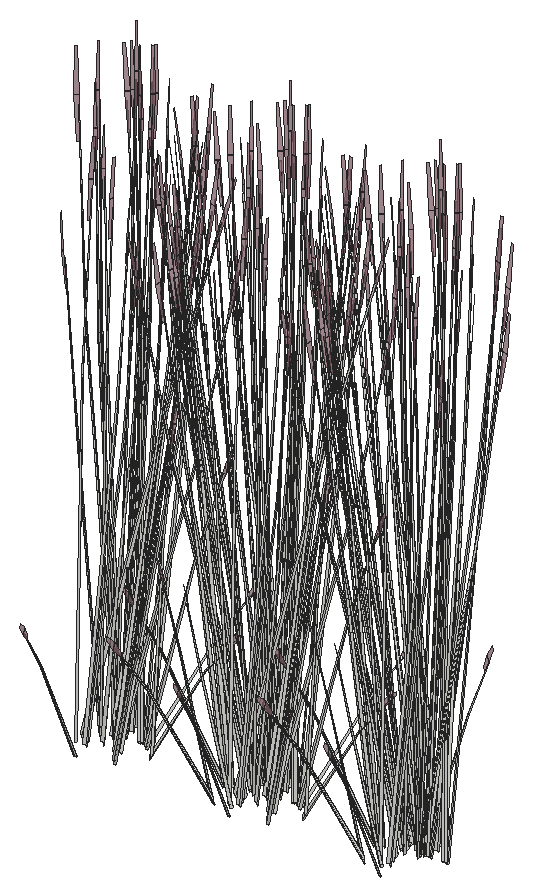
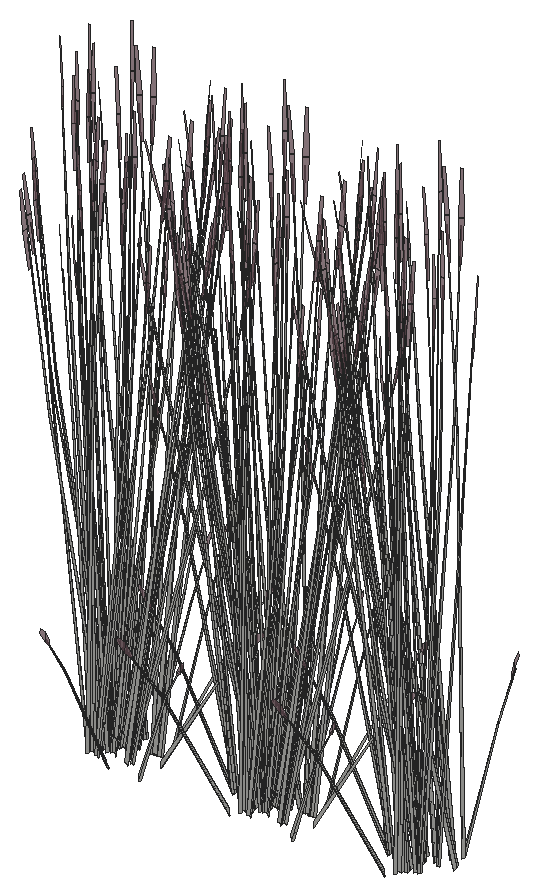
# SketchUp Ruby script. Lengths in inches.
U = 1.inch
M = Sketchup.active_model
def pt(a) = Geom::Point3d.new(a.map { |v| v * U })
def face(e, loops, mat)
  f = e.add_face(loops[0].map { |a| pt(a) })
  loops[1..].each { |l| e.add_face(l.map { |a| pt(a) }).erase! }
  f.material = f.back_material = mat if mat
  f
end
# faces: each face lists its corners as indices into pts; further lists are holes
def faces(e, pts, list, mat = nil) = list.each { |f| face(e, (f[0].is_a?(Array) ? f : [f]).map { |l| l.map { |i| pts[i] } }, mat) }
# xy, xz, yz: faces in a plane at the given z, y or x. An outline is a flat list of corners, or four numbers for a rectangle; further outlines are holes
def ring(l) = l.size == 4 ? [[l[0], l[1]], [l[2], l[1]], [l[2], l[3]], [l[0], l[3]]] : l.each_slice(2).to_a
def flat(e, list, mat, &to3) = list.each { |f| face(e, (f[0].is_a?(Array) ? f : [f]).map { |l| ring(l).map { |u, v| to3.(u, v) } }, mat) }
def xy(e, z, list, mat = nil) = flat(e, list, mat) { |x, y| [x, y, z] }
def xz(e, y, list, mat = nil) = flat(e, list, mat) { |x, z| [x, y, z] }
def yz(e, x, list, mat = nil) = flat(e, list, mat) { |y, z| [x, y, z] }
def lines(e, pts, list) = list.each { |a, b| e.add_line(pt(pts[a]), pt(pts[b])) }
# prism: a flat outline (further loops are holes) pulled along v
def prism(e, loops, v, mat = nil)
  f = face(e, loops, mat); d = Geom::Vector3d.new(v.map { |x| x * U })
  f.pushpull(f.normal.samedirection?(d) ? d.length : -d.length)
end
def box(e, o, s, mat = nil) = prism(e, [[o, [o[0] + s[0], o[1], o[2]], [o[0] + s[0], o[1] + s[1], o[2]], [o[0], o[1] + s[1], o[2]]]], [0, 0, s[2]], mat)
def at(x, y, z, deg = 0) = Geom::Transformation.translation(pt([x, y, z])) * Geom::Transformation.rotation(ORIGIN, Z_AXIS, deg.degrees)
def axes(o, x, y, z) = Geom::Transformation.new([*x, 0, *y, 0, *z, 0, *pt(o).to_a, 1])
def part(name) = M.definitions.add(name)
# library, detail: a bought-in or finely detailed component or shape, given as its bounding box
def library(name, o, s) = part(name).tap { |d| box(d.entities, o, s) }
def detail(e, o, s) = box(e.add_group.entities, o, s)
def put(e, d, t, mat = nil) = e.add_instance(d, t).tap { |i| i.material = mat if mat }
def group(e, t, mat = nil) = e.add_group.tap { |g| g.transformation = t; g.material = mat if mat }.entities
root = M.entities
M.materials.add("LightPink_Translucent").color = [144, 107, 117]
M.materials["LightPink_Translucent"].alpha = 0.75
c1 = part("blade")
p = [[2.15,0.21,22],[0,0.17,0],[0.09,0.45,0],[2.18,0.31,22],[2.29,0.31,22],[0.38,0.45,0],
  [2.48,0.24,33],[2.49,0.24,33],[2.48,0.22,33]]
faces(c1.entities,p,[[0,1,2,3],[4,5,2,3],[6,3,4,7],[8,0,3,6]])
c2 = part("seeds")
p = [[0.3,-0.1,1.38],[-0.01,-0.03,1.59],[-0.01,-0.03,0.03],[0.14,-0.07,-0.07],[0.29,-0.03,3],[0.15,0.01,3.11]]
faces(c2.entities,p,[[0,1,2,3],[1,0,4,5]],"LightPink_Translucent")
c3 = part("blade with seeds")
put(c3.entities,c1,at(0,0,0))
put(c3.entities,c2,axes([2.4,0.25,30.99],[1.5799,-0.05474,1.17369],[-0.12525,1.92788,0.29478],[-0.07173,-0.02425,1.56792]))
put(root,c3,axes([278.62,55.33,257.2],[-0.76598,-0.27433,0],[0.36864,-0.57001,0],[0,0,1.62707]))
put(root,c3,axes([280.39,56.02,257.375],[0.47504,0.61229,0],[-0.79476,0.34146,-0.51607],[-0.18101,0.07777,1.63711]))
put(root,c3,axes([279.42,54.01,257.3],[-0.70674,-0.52593,-0.06131],[0.70717,-0.52625,0],[-0.02468,-0.01837,1.75571]))
put(root,c3,axes([279.8125,55.63,257.33],[0.95122,0.19861,0.30756],[-0.23797,0.7099,-0.36492],[-0.15744,0.08885,1.64885]))
put(root,c3,axes([278.42,50.1875,256.49],[-0.12744,0.02202,1.76342],[-0.70477,-0.24781,-0.26939],[0.01183,-0.2067,0.30037]))
put(root,c3,axes([277.85,53.32,257.21],[0.36864,-0.55059,-0.44739],[0.76598,0.26498,0.21531],[0,-0.12692,1.43643]))
put(root,c3,axes([278.79,55.09,257.2],[-0.24791,-0.5268,0],[0.70791,-0.18448,0],[0,0,1.54371]))
put(root,c3,axes([279.79,54.05,257.21],[-0.36864,0.55059,-0.44739],[-0.76598,-0.26498,0.21531],[0,0.12692,1.43643]))
put(root,c3,axes([279.1875,53.46,257.21],[0,-0.70701,0],[0.95008,0,0],[0,0,1.79456]))
put(root,c3,axes([279.66,53.74,257.29],[0,0.70667,-0.05637],[-0.95008,0,0],[0,0.02221,1.79368]))
put(root,c3,axes([279.21,55.11,257.29],[0.33034,0.70197,-0.06012],[-0.94388,0.24598,0],[0.01154,0.02451,1.72173]))
put(root,c3,axes([277.25,51.35,257.375],[-0.47504,-0.61229,0],[0.79476,-0.34146,-0.51607],[0.18101,-0.07777,1.63711]))
put(root,c3,axes([281.9375,54.19,257.2],[-0.94962,-0.00489,-0.04976],[0,-0.68292,0.49943],[-0.02984,0.15546,1.58352]))
put(root,c3,axes([279.8125,53.89,257.21],[0.53038,0.39469,0],[-0.53038,0.39469,0],[0,0,1.69266]))
put(root,c3,axes([279.49,55.34,257.2],[0.76598,0.27433,0],[-0.36864,0.57001,0],[0,0,1.74954]))
put(root,c3,axes([281.74,54.29,257.03],[-0.53038,0.38124,-0.30978],[-0.53038,-0.38124,0.30978],[0,0.1228,1.38974]))
put(root,c3,axes([280.23,54.22,257.09],[0.2786,0.55945,-0.69212],[-0.80253,0.20149,-0.18165],[0.03079,0.18945,1.52773]))
put(root,c3,axes([279.83,53.62,257.21],[0.85008,0,0],[0,0.63259,0],[0,0,1.78407]))
put(root,c3,axes([278.18,53.04,257.67],[-0.08854,-0.69723,-0.29095],[0.92215,-0.04216,-0.50002],[0.16238,-0.09287,1.59708]))
put(root,c3,axes([279.88,53.6,257.67],[0.85568,0.29155,-0.29095],[-0.41201,0.61537,-0.50002],[0.02689,0.15109,1.59708]))
put(root,c3,axes([278.0625,51.5,257.03],[0.70886,0.15119,-0.30978],[-0.17848,0.53243,0.30978],[0.1429,-0.0614,1.38974]))
put(root,c3,axes([282.11,54.3,257.02],[0,0.61104,-0.49651],[-0.85008,0,0],[0,0.13917,1.57504]))
put(root,c3,axes([277.9,51.26,257.02],[0.7111,-0.30552,-0.49651],[0.42504,0.54784,0],[0.16196,-0.06958,1.57504]))
put(root,c3,axes([279.72,55.02,257.18],[0.79769,-0.20732,-0.19198],[0.2803,0.59721,0.00008],[0.08805,-0.02292,1.73897]))
put(root,c3,axes([279.73,53.24,257.21],[0.45644,0.51287,-0.44739],[-0.69137,0.36116,0.21531],[0.14771,0.06346,1.43643]))
put(root,c3,axes([278.74,52.51,257.06],[0.51177,-0.45928,-0.62353],[0.63575,0.41646,-0.16365],[0.20507,-0.11457,1.37633]))
put(root,c3,axes([280.98,52.1,257.03],[0.17848,0.53243,-0.30978],[-0.70886,0.15119,0.30978],[0.1429,0.0614,1.38974]))
put(root,c3,axes([282.32,53.84,257.375],[0.95008,0,0],[0,0.68292,-0.51607],[0,0.15554,1.63711]))
put(root,c3,axes([279.25,52.95,257.67],[0.76714,-0.40567,-0.29095],[0.51013,0.57321,-0.50002],[0.18927,0.05821,1.59708]))
put(root,c3,axes([277.3125,52.59,256.59],[-0.74787,0.24464,1.28929],[-0.23804,-0.70192,0.50096],[0.45924,0.01168,1.46642]))
put(root,c3,axes([280.75,51.51,257.375],[0.47504,-0.61229,0],[0.79476,0.34146,-0.51607],[0.18101,0.07777,1.63711]))
put(root,c3,axes([281.54,51.24,256.49],[-0.11372,-0.04814,1.76342],[-0.29211,-0.53779,-0.26939],[0.19706,-0.14594,0.30037]))
put(root,c3,axes([281.18,51.875,257.02],[0.7111,0.30552,-0.49651],[-0.42504,0.54784,0],[0.16196,0.06958,1.57504]))
put(root,c3,axes([281.15,56.22,256.49],[0.05536,-0.08822,1.76342],[0.69692,-0.25981,-0.26939],[0.21129,0.13447,0.30037]))
put(root,c3,axes([280.14,53.05,257.06],[0.79037,0.10018,-0.62353],[-0.16679,0.61794,-0.16365],[0.23587,0.07488,1.37633]))
put(root,c3,axes([283.51,53.41,257.26],[-0.47106,-0.39072,-0.06488],[0.51591,-0.35801,-0.29416],[0.14618,-0.02521,0.97024]))
put(root,c3,axes([290.68,53.45,256.49],[0.01927,0.0963,1.76342],[-0.38846,0.5029,-0.26939],[-0.27592,-0.02535,0.30037]))
put(root,c3,axes([290.47,56.15,256.49],[0.10192,0.06105,1.76342],[0.17281,0.56562,-0.26939],[-0.22588,0.12062,0.30037]))
put(root,c3,axes([293.22,54.32,257.06],[-0.79037,-0.10018,-0.62353],[0.16679,-0.61794,-0.16365],[-0.23587,-0.07488,1.37633]))
put(root,c3,axes([282.62,53.93,256.98],[-0.48937,0.07333,1.41583],[-0.07789,-0.58369,0.08104],[0.34275,-0.08835,0.80566]))
put(root,c3,axes([283.15,53.55,256.49],[-0.03971,-0.09277,1.76342],[0.27541,-0.54264,-0.26939],[0.27782,-0.00781,0.30037]))
put(root,c3,axes([292.1875,55.49,257.02],[-0.7111,-0.30552,-0.49651],[0.42504,-0.54784,0],[-0.16196,-0.06958,1.57504]))
put(root,c3,axes([291.875,50.94,256.49],[-0.0736,0.08049,1.76342],[-0.74378,0.17355,-0.26939],[-0.17968,-0.15788,0.30037]))
put(root,c3,axes([292.62,55.86,257.375],[-0.47504,0.61229,0],[-0.79476,-0.34146,-0.51607],[-0.18101,-0.07777,1.63711]))
put(root,c3,axes([291.41,51.25,257.13],[-0.21918,0.49894,-0.03893],[-0.6746,-0.15348,-0.17649],[-0.10242,-0.08161,0.58215]))
put(root,c3,axes([294.12,54.42,257.67],[-0.76714,0.40567,-0.29095],[-0.51013,-0.57321,-0.50002],[-0.18927,-0.05821,1.59708]))
put(root,c3,axes([291.05,53.53,257.375],[-0.95008,0,0],[0,-0.68292,-0.51607],[0,-0.15554,1.63711]))
put(root,c3,axes([292.38,55.27,257.03],[-0.17848,-0.53243,-0.30978],[0.70886,-0.15119,0.30978],[-0.1429,-0.0614,1.38974]))
put(root,c3,axes([294.63,54.86,257.06],[-0.51177,0.45928,-0.62353],[-0.63575,-0.41646,-0.16365],[-0.20507,0.11457,1.37633]))
put(root,c3,axes([291.79,53.35,257.33],[-0.70674,0.51372,0.30756],[-0.70717,-0.50832,-0.36492],[-0.02468,-0.14589,1.64885]))
put(root,c3,axes([294.98,54.6,257.46],[-0.74193,-0.49181,-0.25192],[0.6243,-0.55226,0.5513],[-0.19979,0.05753,1.68216]))
put(root,c3,axes([293.63,54.13,257.21],[-0.45644,-0.51287,-0.44739],[0.69137,-0.36116,0.21531],[-0.14771,-0.06346,1.43643]))
put(root,c3,axes([294.61,54.5,257.21],[-0.82508,0.03772,-0.44739],[-0.07462,-0.62614,0.21531],[-0.14771,0.06346,1.43643]))
put(root,c3,axes([293.7,54.42,257.4375],[0.20138,-0.72405,-0.23429],[0.95485,0.12621,0.51271],[-0.16685,-0.09999,1.5644]))
put(root,c3,axes([295.47,56.11,257.02],[-0.7111,0.30552,-0.49651],[-0.42504,-0.54784,0],[-0.16196,0.06958,1.57504]))
put(root,c3,axes([291.26,53.07,257.02],[0,-0.61104,-0.49651],[0.85008,0,0],[0,-0.13917,1.57504]))
put(root,c3,axes([295.52,55.95,257.19],[-0.46912,-0.61443,-0.05142],[0.79476,-0.34146,0.51607],[-0.19584,0.0585,1.6363]))
put(root,c3,axes([295.31,55.87,257.03],[-0.70886,-0.15119,-0.30978],[0.17848,-0.53243,0.30978],[-0.1429,0.0614,1.38974]))
put(root,c3,axes([293.48,53.77,257.67],[-0.85568,-0.29155,-0.29095],[0.41201,-0.61537,-0.50002],[-0.02689,-0.15109,1.59708]))
put(root,c3,axes([295.18,54.33,257.67],[0.08854,0.69723,-0.29095],[-0.92215,0.04216,-0.50002],[-0.16238,0.09287,1.59708]))
put(root,c3,axes([293.1,53.15,257.1],[-0.31203,-0.62659,-0.69835],[0.89884,-0.22566,-0.18329],[-0.03449,-0.21218,1.54149]))
put(root,c3,axes([291.625,53.08,257.03],[0.53038,-0.38124,-0.30978],[0.53038,0.38124,0.30978],[0,-0.1228,1.38974]))
put(root,c3,axes([294.02,50.62,257.13],[-0.52505,0.35054,-0.03893],[-0.48109,-0.38392,-0.17649],[-0.03387,-0.10878,0.58215]))
put(root,c3,axes([294.34,55.33,257.2],[-0.76598,-0.27433,0],[0.36864,-0.57001,0],[0,0,1.62707]))
put(root,c3,axes([296.12,56.02,257.375],[0.47504,0.61229,0],[-0.79476,0.34146,-0.51607],[-0.18101,0.07777,1.63711]))
put(root,c3,axes([295.15,54.01,257.3],[-0.70674,-0.52593,-0.06131],[0.70717,-0.52625,0],[-0.02468,-0.01837,1.75571]))
put(root,c3,axes([295.54,55.63,257.33],[0.95122,0.19861,0.30756],[-0.23797,0.7099,-0.36492],[-0.15744,0.08885,1.64885]))
put(root,c3,axes([294.15,50.1875,256.49],[-0.12744,0.02202,1.76342],[-0.70477,-0.24781,-0.26939],[0.01183,-0.2067,0.30037]))
put(root,c3,axes([293.58,53.32,257.21],[0.36864,-0.55059,-0.44739],[0.76598,0.26498,0.21531],[0,-0.12692,1.43643]))
put(root,c3,axes([294.52,55.09,257.2],[-0.24791,-0.5268,0],[0.70791,-0.18448,0],[0,0,1.54371]))
put(root,c3,axes([295.52,54.05,257.21],[-0.36864,0.55059,-0.44739],[-0.76598,-0.26498,0.21531],[0,0.12692,1.43643]))
put(root,c3,axes([294.92,53.46,257.21],[0,-0.70701,0],[0.95008,0,0],[0,0,1.79456]))
put(root,c3,axes([295.39,53.74,257.29],[0,0.70667,-0.05637],[-0.95008,0,0],[0,0.02221,1.79368]))
put(root,c3,axes([294.9375,55.11,257.29],[0.33034,0.70197,-0.06012],[-0.94388,0.24598,0],[0.01154,0.02451,1.72173]))
put(root,c3,axes([292.98,51.35,257.375],[-0.47504,-0.61229,0],[0.79476,-0.34146,-0.51607],[0.18101,-0.07777,1.63711]))
put(root,c3,axes([297.67,54.19,257.2],[-0.94962,-0.00489,-0.04976],[0,-0.68292,0.49943],[-0.02984,0.15546,1.58352]))
put(root,c3,axes([295.54,53.89,257.21],[0.53038,0.39469,0],[-0.53038,0.39469,0],[0,0,1.69266]))
put(root,c3,axes([295.21,55.34,257.2],[0.76598,0.27433,0],[-0.36864,0.57001,0],[0,0,1.74954]))
put(root,c3,axes([297.47,54.29,257.03],[-0.53038,0.38124,-0.30978],[-0.53038,-0.38124,0.30978],[0,0.1228,1.38974]))
put(root,c3,axes([295.95,54.22,257.09],[0.2786,0.55945,-0.69212],[-0.80253,0.20149,-0.18165],[0.03079,0.18945,1.52773]))
put(root,c3,axes([295.56,53.62,257.21],[0.85008,0,0],[0,0.63259,0],[0,0,1.78407]))
put(root,c3,axes([293.91,53.04,257.67],[-0.08854,-0.69723,-0.29095],[0.92215,-0.04216,-0.50002],[0.16238,-0.09287,1.59708]))
put(root,c3,axes([295.61,53.6,257.67],[0.85568,0.29155,-0.29095],[-0.41201,0.61537,-0.50002],[0.02689,0.15109,1.59708]))
put(root,c3,axes([293.79,51.5,257.03],[0.70886,0.15119,-0.30978],[-0.17848,0.53243,0.30978],[0.1429,-0.0614,1.38974]))
put(root,c3,axes([297.83,54.3,257.02],[0,0.61104,-0.49651],[-0.85008,0,0],[0,0.13917,1.57504]))
put(root,c3,axes([293.625,51.26,257.02],[0.7111,-0.30552,-0.49651],[0.42504,0.54784,0],[0.16196,-0.06958,1.57504]))
put(root,c3,axes([295.45,55.02,257.18],[0.79769,-0.20732,-0.19198],[0.2803,0.59721,0.00008],[0.08805,-0.02292,1.73897]))
put(root,c3,axes([295.46,53.24,257.21],[0.45644,0.51287,-0.44739],[-0.69137,0.36116,0.21531],[0.14771,0.06346,1.43643]))
put(root,c3,axes([294.47,52.51,257.06],[0.51177,-0.45928,-0.62353],[0.63575,0.41646,-0.16365],[0.20507,-0.11457,1.37633]))
put(root,c3,axes([296.71,52.1,257.03],[0.17848,0.53243,-0.30978],[-0.70886,0.15119,0.30978],[0.1429,0.0614,1.38974]))
put(root,c3,axes([298.05,53.84,257.375],[0.95008,0,0],[0,0.68292,-0.51607],[0,0.15554,1.63711]))
put(root,c3,axes([294.98,52.95,257.67],[0.76714,-0.40567,-0.29095],[0.51013,0.57321,-0.50002],[0.18927,0.05821,1.59708]))
put(root,c3,axes([293.04,52.59,256.59],[-0.74787,0.24464,1.28929],[-0.23804,-0.70192,0.50096],[0.45924,0.01168,1.46642]))
put(root,c3,axes([296.48,51.51,257.375],[0.47504,-0.61229,0],[0.79476,0.34146,-0.51607],[0.18101,0.07777,1.63711]))
put(root,c3,axes([297.27,51.24,256.49],[-0.11372,-0.04814,1.76342],[-0.29211,-0.53779,-0.26939],[0.19706,-0.14594,0.30037]))
put(root,c3,axes([296.91,51.875,257.02],[0.7111,0.30552,-0.49651],[-0.42504,0.54784,0],[0.16196,0.06958,1.57504]))
put(root,c3,axes([296.875,56.22,256.49],[0.05536,-0.08822,1.76342],[0.69692,-0.25981,-0.26939],[0.21129,0.13447,0.30037]))
put(root,c3,axes([306.13,53.45,256.49],[0.01927,0.0963,1.76342],[-0.38846,0.5029,-0.26939],[-0.27592,-0.02535,0.30037]))
put(root,c3,axes([295.87,53.05,257.06],[0.79037,0.10018,-0.62353],[-0.16679,0.61794,-0.16365],[0.23587,0.07488,1.37633]))
put(root,c3,axes([299.24,53.41,257.26],[-0.47106,-0.39072,-0.06488],[0.51591,-0.35801,-0.29416],[0.14618,-0.02521,0.97024]))
put(root,c3,axes([305.92,56.15,256.49],[0.10192,0.06105,1.76342],[0.17281,0.56562,-0.26939],[-0.22588,0.12062,0.30037]))
put(root,c3,axes([308.67,54.32,257.06],[-0.79037,-0.10018,-0.62353],[0.16679,-0.61794,-0.16365],[-0.23587,-0.07488,1.37633]))
put(root,c3,axes([307.63,55.49,257.02],[-0.7111,-0.30552,-0.49651],[0.42504,-0.54784,0],[-0.16196,-0.06958,1.57504]))
put(root,c3,axes([307.32,50.94,256.49],[-0.0736,0.08049,1.76342],[-0.74378,0.17355,-0.26939],[-0.17968,-0.15788,0.30037]))
put(root,c3,axes([298.35,53.93,256.98],[-0.48937,0.07333,1.41583],[-0.07789,-0.58369,0.08104],[0.34275,-0.08835,0.80566]))
put(root,c3,axes([298.88,53.55,256.49],[-0.03971,-0.09277,1.76342],[0.27541,-0.54264,-0.26939],[0.27782,-0.00781,0.30037]))
put(root,c3,axes([308.07,55.86,257.375],[-0.47504,0.61229,0],[-0.79476,-0.34146,-0.51607],[-0.18101,-0.07777,1.63711]))
put(root,c3,axes([306.86,51.25,257.13],[-0.21918,0.49894,-0.03893],[-0.6746,-0.15348,-0.17649],[-0.10242,-0.08161,0.58215]))
put(root,c3,axes([309.57,54.42,257.67],[-0.76714,0.40567,-0.29095],[-0.51013,-0.57321,-0.50002],[-0.18927,-0.05821,1.59708]))
put(root,c3,axes([306.5,53.53,257.375],[-0.95008,0,0],[0,-0.68292,-0.51607],[0,-0.15554,1.63711]))
put(root,c3,axes([307.83,55.27,257.03],[-0.17848,-0.53243,-0.30978],[0.70886,-0.15119,0.30978],[-0.1429,-0.0614,1.38974]))
put(root,c3,axes([310.08,54.86,257.06],[-0.51177,0.45928,-0.62353],[-0.63575,-0.41646,-0.16365],[-0.20507,0.11457,1.37633]))
put(root,c3,axes([307.23,53.35,257.33],[-0.70674,0.51372,0.30756],[-0.70717,-0.50832,-0.36492],[-0.02468,-0.14589,1.64885]))
put(root,c3,axes([310.43,54.6,257.46],[-0.74193,-0.49181,-0.25192],[0.6243,-0.55226,0.5513],[-0.19979,0.05753,1.68216]))
put(root,c3,axes([309.08,54.13,257.21],[-0.45644,-0.51287,-0.44739],[0.69137,-0.36116,0.21531],[-0.14771,-0.06346,1.43643]))
put(root,c3,axes([310.05,54.5,257.21],[-0.82508,0.03772,-0.44739],[-0.07462,-0.62614,0.21531],[-0.14771,0.06346,1.43643]))
put(root,c3,axes([309.15,54.42,257.4375],[0.20138,-0.72405,-0.23429],[0.95485,0.12621,0.51271],[-0.16685,-0.09999,1.5644]))
put(root,c3,axes([310.92,56.11,257.02],[-0.7111,0.30552,-0.49651],[-0.42504,-0.54784,0],[-0.16196,0.06958,1.57504]))
put(root,c3,axes([306.71,53.07,257.02],[0,-0.61104,-0.49651],[0.85008,0,0],[0,-0.13917,1.57504]))
put(root,c3,axes([310.97,55.95,257.19],[-0.46912,-0.61443,-0.05142],[0.79476,-0.34146,0.51607],[-0.19584,0.0585,1.6363]))
put(root,c3,axes([310.75,55.87,257.03],[-0.70886,-0.15119,-0.30978],[0.17848,-0.53243,0.30978],[-0.1429,0.0614,1.38974]))
put(root,c3,axes([308.93,53.77,257.67],[-0.85568,-0.29155,-0.29095],[0.41201,-0.61537,-0.50002],[-0.02689,-0.15109,1.59708]))
put(root,c3,axes([310.63,54.33,257.67],[0.08854,0.69723,-0.29095],[-0.92215,0.04216,-0.50002],[-0.16238,0.09287,1.59708]))
put(root,c3,axes([308.55,53.15,257.1],[-0.31203,-0.62659,-0.69835],[0.89884,-0.22566,-0.18329],[-0.03449,-0.21218,1.54149]))
put(root,c3,axes([307.07,53.08,257.03],[0.53038,-0.38124,-0.30978],[0.53038,0.38124,0.30978],[0,-0.1228,1.38974]))
put(root,c3,axes([309.47,50.62,257.13],[-0.52505,0.35054,-0.03893],[-0.48109,-0.38392,-0.17649],[-0.03387,-0.10878,0.58215]))
put(root,c3,axes([309.79,55.33,257.2],[-0.76598,-0.27433,0],[0.36864,-0.57001,0],[0,0,1.62707]))
put(root,c3,axes([311.57,56.02,257.375],[0.47504,0.61229,0],[-0.79476,0.34146,-0.51607],[-0.18101,0.07777,1.63711]))
put(root,c3,axes([310.6,54.01,257.3],[-0.70674,-0.52593,-0.06131],[0.70717,-0.52625,0],[-0.02468,-0.01837,1.75571]))
put(root,c3,axes([310.99,55.63,257.33],[0.95122,0.19861,0.30756],[-0.23797,0.7099,-0.36492],[-0.15744,0.08885,1.64885]))
put(root,c3,axes([309.6,50.1875,256.49],[-0.12744,0.02202,1.76342],[-0.70477,-0.24781,-0.26939],[0.01183,-0.2067,0.30037]))
put(root,c3,axes([309.02,53.32,257.21],[0.36864,-0.55059,-0.44739],[0.76598,0.26498,0.21531],[0,-0.12692,1.43643]))
put(root,c3,axes([309.97,55.09,257.2],[-0.24791,-0.5268,0],[0.70791,-0.18448,0],[0,0,1.54371]))
put(root,c3,axes([309.07,56.2,256.49],[0.12297,-0.03325,1.76342],[0.73967,0.18301,-0.26939],[0.02163,0.20626,0.30037]))
put(root,c3,axes([310.97,54.05,257.21],[-0.36864,0.55059,-0.44739],[-0.76598,-0.26498,0.21531],[0,0.12692,1.43643]))
put(root,c3,axes([310.36,53.46,257.21],[0,-0.70701,0],[0.95008,0,0],[0,0,1.79456]))
put(root,c3,axes([310.84,53.74,257.29],[0,0.70667,-0.05637],[-0.95008,0,0],[0,0.02221,1.79368]))
put(root,c3,axes([310.39,55.11,257.29],[0.33034,0.70197,-0.06012],[-0.94388,0.24598,0],[0.01154,0.02451,1.72173]))
put(root,c3,axes([308.43,51.35,257.375],[-0.47504,-0.61229,0],[0.79476,-0.34146,-0.51607],[0.18101,-0.07777,1.63711]))
put(root,c3,axes([313.11,54.19,257.2],[-0.94962,-0.00489,-0.04976],[0,-0.68292,0.49943],[-0.02984,0.15546,1.58352]))
put(root,c3,axes([310.99,53.89,257.21],[0.53038,0.39469,0],[-0.53038,0.39469,0],[0,0,1.69266]))
put(root,c3,axes([310.66,55.34,257.2],[0.76598,0.27433,0],[-0.36864,0.57001,0],[0,0,1.74954]))
put(root,c3,axes([312.92,54.29,257.03],[-0.53038,0.38124,-0.30978],[-0.53038,-0.38124,0.30978],[0,0.1228,1.38974]))
put(root,c3,axes([311.4,54.22,257.09],[0.2786,0.55945,-0.69212],[-0.80253,0.20149,-0.18165],[0.03079,0.18945,1.52773]))
put(root,c3,axes([311.01,53.62,257.21],[0.85008,0,0],[0,0.63259,0],[0,0,1.78407]))
put(root,c3,axes([309.36,53.04,257.67],[-0.08854,-0.69723,-0.29095],[0.92215,-0.04216,-0.50002],[0.16238,-0.09287,1.59708]))
put(root,c3,axes([311.06,53.6,257.67],[0.85568,0.29155,-0.29095],[-0.41201,0.61537,-0.50002],[0.02689,0.15109,1.59708]))
put(root,c3,axes([309.24,51.5,257.03],[0.70886,0.15119,-0.30978],[-0.17848,0.53243,0.30978],[0.1429,-0.0614,1.38974]))
put(root,c3,axes([313.28,54.3,257.02],[0,0.61104,-0.49651],[-0.85008,0,0],[0,0.13917,1.57504]))
put(root,c3,axes([309.07,51.26,257.02],[0.7111,-0.30552,-0.49651],[0.42504,0.54784,0],[0.16196,-0.06958,1.57504]))
put(root,c3,axes([310.9,55.02,257.18],[0.79769,-0.20732,-0.19198],[0.2803,0.59721,0.00008],[0.08805,-0.02292,1.73897]))
put(root,c3,axes([310.91,53.24,257.21],[0.45644,0.51287,-0.44739],[-0.69137,0.36116,0.21531],[0.14771,0.06346,1.43643]))
